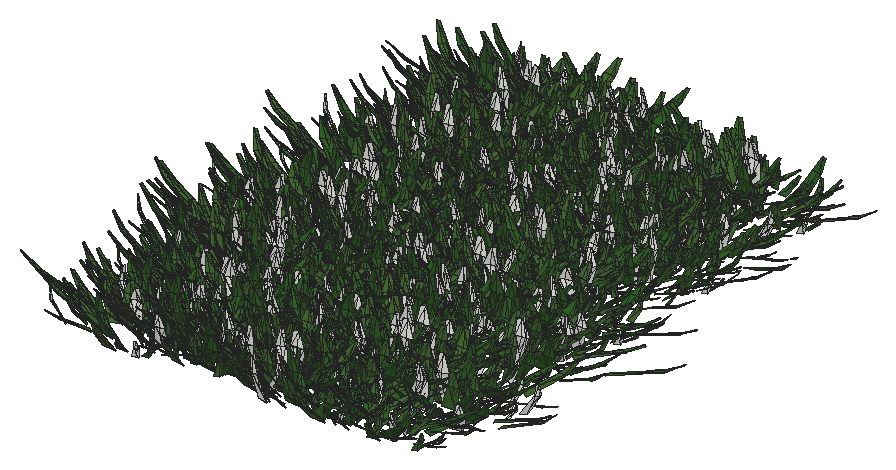
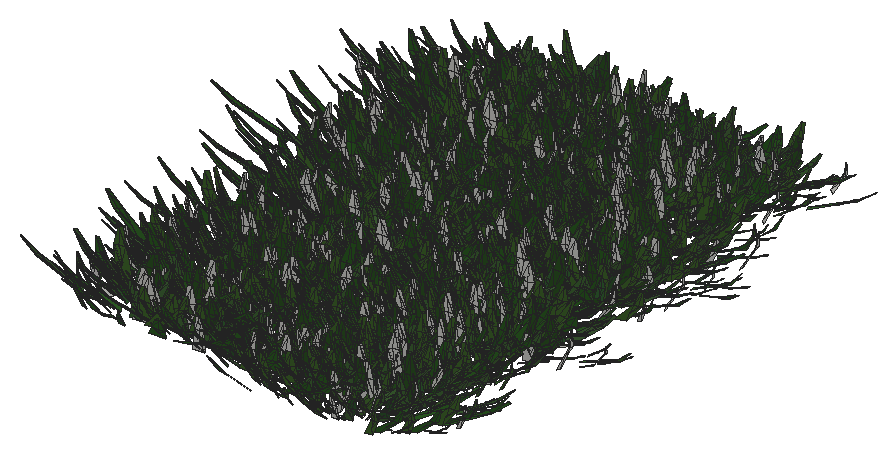
# SketchUp Ruby script. Lengths in inches.
U = 1.inch
M = Sketchup.active_model
def pt(a) = Geom::Point3d.new(a.map { |v| v * U })
def face(e, loops, mat)
  f = e.add_face(loops[0].map { |a| pt(a) })
  loops[1..].each { |l| e.add_face(l.map { |a| pt(a) }).erase! }
  f.material = f.back_material = mat if mat
  f
end
# faces: each face lists its corners as indices into pts; further lists are holes
def faces(e, pts, list, mat = nil) = list.each { |f| face(e, (f[0].is_a?(Array) ? f : [f]).map { |l| l.map { |i| pts[i] } }, mat) }
# xy, xz, yz: faces in a plane at the given z, y or x. An outline is a flat list of corners, or four numbers for a rectangle; further outlines are holes
def ring(l) = l.size == 4 ? [[l[0], l[1]], [l[2], l[1]], [l[2], l[3]], [l[0], l[3]]] : l.each_slice(2).to_a
def flat(e, list, mat, &to3) = list.each { |f| face(e, (f[0].is_a?(Array) ? f : [f]).map { |l| ring(l).map { |u, v| to3.(u, v) } }, mat) }
def xy(e, z, list, mat = nil) = flat(e, list, mat) { |x, y| [x, y, z] }
def xz(e, y, list, mat = nil) = flat(e, list, mat) { |x, z| [x, y, z] }
def yz(e, x, list, mat = nil) = flat(e, list, mat) { |y, z| [x, y, z] }
def lines(e, pts, list) = list.each { |a, b| e.add_line(pt(pts[a]), pt(pts[b])) }
# prism: a flat outline (further loops are holes) pulled along v
def prism(e, loops, v, mat = nil)
  f = face(e, loops, mat); d = Geom::Vector3d.new(v.map { |x| x * U })
  f.pushpull(f.normal.samedirection?(d) ? d.length : -d.length)
end
def box(e, o, s, mat = nil) = prism(e, [[o, [o[0] + s[0], o[1], o[2]], [o[0] + s[0], o[1] + s[1], o[2]], [o[0], o[1] + s[1], o[2]]]], [0, 0, s[2]], mat)
def at(x, y, z, deg = 0) = Geom::Transformation.translation(pt([x, y, z])) * Geom::Transformation.rotation(ORIGIN, Z_AXIS, deg.degrees)
def axes(o, x, y, z) = Geom::Transformation.new([*x, 0, *y, 0, *z, 0, *pt(o).to_a, 1])
def part(name) = M.definitions.add(name)
# library, detail: a bought-in or finely detailed component or shape, given as its bounding box
def library(name, o, s) = part(name).tap { |d| box(d.entities, o, s) }
def detail(e, o, s) = box(e.add_group.entities, o, s)
def put(e, d, t, mat = nil) = e.add_instance(d, t).tap { |i| i.material = mat if mat }
def group(e, t, mat = nil) = e.add_group.tap { |g| g.transformation = t; g.material = mat if mat }.entities
root = M.entities
M.materials.add("Material82").color = [68, 110, 58]
M.materials.add("Material83").color = [48, 90, 38]
M.materials.add("Material84").color = [68, 110, 48]
M.materials.add("Material85").color = [48, 90, 48]
M.materials.add("Material86").color = [58, 110, 58]
M.materials.add("Material87").color = [58, 90, 38]
M.materials.add("Material88").color = [68, 100, 58]
M.materials.add("Material89").color = [48, 100, 38]
c1 = part("grass00")
p = [[-0.6875,0.15,0],[-0.56,0.08,5.52],[-0.04,0.03,2.76],[0.48,-0.02,0],[0.35,-0.02,5.52],[-0.1,-0.14,5.52],
  [-0.12,0.65,8.37],[-0.42,0.65,8.37]]
faces(c1.entities,p,[[0,1,2,3],[3,2,4],[1,5,2],[5,4,2],[1,6,5],[4,5,6],[7,6,1]])
c2 = part("Group16\#1")
put(c2.entities,c1,axes([1.44,-0.61,-0.01],[0.05352,0.12609,0],[-0.10704,0.04543,0.07239],[0.06664,-0.02828,0.11628]),"Material85")
put(c2.entities,c1,axes([0.76,-0.15,-0.01],[0.04676,0.24062,0],[-0.23162,0.04501,0.06642],[0.0652,-0.01267,0.23595]),"Material82")
put(c2.entities,c1,axes([0.79,0.01,-0.01],[-0.00606,0.34651,0],[-0.34381,-0.00602,0.0432],[0.04319,0.00076,0.34386]))
put(c2.entities,c1,axes([1,0.23,-0.01],[-0.07192,0.31144,0],[-0.28722,-0.06632,0.1236],[0.12043,0.02781,0.29478]),"Material84")
put(c2.entities,c1,axes([1.66,0.77,-0.01],[-0.13828,0.29651,0],[-0.21551,-0.1005,0.22471],[0.20365,0.09498,0.23779]),"Material89")
put(c2.entities,c1,axes([0.6875,0.52,-0.01],[-0.18126,0.24051,0],[-0.22746,-0.17142,0.09788],[0.07817,0.05891,0.28481]),"Material84")
put(c2.entities,c1,axes([0.68,0.78,-0.01],[-0.215,0.18688,0],[-0.12385,-0.14248,0.21334],[0.13995,0.16101,0.18878]),"Material82")
put(c2.entities,c1,axes([0.56,1,-0.01],[-0.13756,0.07624,0],[-0.06159,-0.11112,0.0927],[0.04494,0.08108,0.12705]),"Material84")
put(c2.entities,c1,axes([0.2,0.64,-0.01],[-0.23729,0.07254,0],[-0.05711,-0.18681,0.153],[0.04473,0.14632,0.19535]),"Material89")
put(c2.entities,c1,axes([0.0625,0.72,-0.01],[-0.28874,0.02525,0],[-0.02179,-0.24916,0.14647],[0.01276,0.14591,0.25012]),"Material82")
put(c2.entities,c1,axes([-0.08,0.62,-0.01],[-0.34089,-0.04187,0],[0.03255,-0.26504,0.216],[-0.02633,0.21439,0.26703]),"Material89")
put(c2.entities,c1,axes([-0.34,0.98,-0.01],[-0.14314,-0.0493,0],[0.04397,-0.12769,0.06843],[-0.02228,0.0647,0.13505]),"Material89")
put(c2.entities,c1,axes([-0.87,1.45,-0.01],[-0.23488,-0.14114,0],[0.13761,-0.22901,0.06087],[-0.03135,0.05217,0.26717]))
put(c2.entities,c1,axes([-0.72,0.77,-0.01],[-0.14208,-0.13251,0],[0.07209,-0.0773,0.16301],[-0.11118,0.11922,0.1057]),"Material89")
put(c2.entities,c1,axes([-0.62,0.43,-0.01],[-0.14845,-0.21203,0],[0.18654,-0.13061,0.12304],[-0.10079,0.07057,0.22772]),"Material82")
put(c2.entities,c1,axes([-0.68,0.29,-0.01],[-0.13639,-0.32136,0],[0.31723,-0.13464,0.05579],[-0.05136,0.0218,0.34462]),"Material83")
put(c2.entities,c1,axes([-0.64,0.125,-0.01],[-0.0458,-0.23569,0],[0.22124,-0.043,0.08276],[-0.08124,0.01579,0.22538]),"Material86")
put(c2.entities,c1,axes([-1.6,-0.03,-0.01],[0.00576,-0.32897,0],[0.27526,0.00482,0.18018],[-0.18015,-0.00315,0.2753]),"Material84")
put(c2.entities,c1,axes([-1.36,-0.31,-0.01],[0.05718,-0.24765,0],[0.18172,0.04196,0.17267],[-0.16825,-0.03885,0.1865]),"Material89")
put(c2.entities,c1,axes([-1.54,-0.72,-0.01],[0.06537,-0.14017,0],[0.13555,0.06321,0.03939],[-0.0357,-0.01665,0.14956]))
put(c2.entities,c1,axes([-1.19,-0.9,-0.01],[0.09597,-0.12735,0],[0.11214,0.08451,0.07557],[-0.06035,-0.04548,0.14042]),"Material88")
put(c2.entities,c1,axes([-0.47,-0.54,-0.01],[0.11588,-0.10072,0],[0.0618,0.0711,0.12124],[-0.07953,-0.0915,0.0942]))
put(c2.entities,c1,axes([-0.47,-0.84,-0.01],[0.11927,-0.0661,0],[0.06603,0.11913,0.00646],[-0.00313,-0.00565,0.13621]),"Material84")
put(c2.entities,c1,axes([-0.38,-1.24,-0.01],[0.28037,-0.08571,0],[0.0618,0.20215,0.20315],[-0.05939,-0.19428,0.21139]),"Material88")
put(c2.entities,c1,axes([-0.06,-0.66,-0.01],[0.22719,-0.01987,0],[0.01247,0.14255,0.17758],[-0.01547,-0.17691,0.1431]),"Material87")
put(c2.entities,c1,axes([0.11,-0.89,-0.01],[0.14882,0.01828,0],[-0.01058,0.08611,0.12229],[0.01491,-0.12138,0.08676]),"Material85")
put(c2.entities,c1,axes([0.25,-0.72,-0.01],[0.20481,0.07053,0],[-0.06206,0.18022,0.10291],[0.03351,-0.0973,0.1906]),"Material85")
put(c2.entities,c1,axes([0.85,-1.42,-0.01],[0.16481,0.09904,0],[-0.09472,0.15762,0.05616],[0.02893,-0.04814,0.18389]),"Material84")
put(c2.entities,c1,axes([1.01,-1.09,-0.01],[0.21858,0.20385,0],[-0.17495,0.1876,0.15339],[0.10462,-0.11218,0.25652]),"Material89")
put(c2.entities,c1,axes([1.01,-0.71,-0.01],[0.08733,0.12473,0],[-0.06445,0.04512,0.13037],[0.1068,-0.07477,0.07867]),"Material85")
c3 = part("Group15\#1")
put(c3.entities,c2,at(0,0,0))
c4 = part("3darcstudiotree_grass00\#1")
put(c4.entities,c3,at(0,0,0))
put(root,c4,axes([655.18,1033.95,-29.74],[4.10302,-0.30694,0],[0.8385,1.74326,-0.00778],[0.00611,0.0127,1.42033]))
put(root,c4,axes([655.57,1017.02,-29.74],[-2.0309,1.41107,0],[-3.96455,-0.88745,-0.03094],[-0.10652,-0.02384,1.35284]))
put(root,c4,axes([655.39,1018.32,-29.74],[3.97679,-0.10087,0],[0.2922,1.7917,-0.04097],[0.01281,0.07857,1.66267]))
put(root,c4,axes([656.06,1024.5,-29.74],[2.96266,-0.9536,0],[2.21709,1.07131,-0.03627],[0.16479,0.07963,1.88825]))
put(root,c4,axes([657.22,1009.61,-29.74],[-2.64678,-1.36079,0],[3.05956,-0.92555,-0.03114],[0.16031,-0.04849,1.87535]))
put(root,c4,axes([656.63,1048.64,-29.74],[2.77032,-1.11765,0],[2.79461,1.07735,-0.00015],[0.00071,0.00027,1.98495]))
put(root,c4,axes([655.75,1012.55,-29.74],[1.36747,1.27936,0],[-3.91602,0.651,-0.04214],[-0.23603,0.03924,1.93625]))
put(root,c4,axes([657.62,1031.41,-29.74],[-0.46652,-1.63259,0],[3.80254,-0.169,-0.02839],[0.12966,-0.00576,1.31807]))
put(root,c4,axes([657.72,1038.09,-29.74],[-2.24585,-1.17679,0],[2.75058,-0.81643,-0.02546],[0.1532,-0.04547,1.94365]))
put(root,c4,axes([658.32,1047.5,-29.74],[-3.1613,-1.38915,0],[3.20855,-1.13563,-0.02493],[0.08224,-0.02911,1.43253]))
put(root,c4,axes([658.0625,1051.55,-29.74],[-4.11217,-0.39094,0],[0.86082,-1.40827,-0.01967],[0.02693,-0.04406,1.60841]))
put(root,c4,axes([657.42,1021.11,-29.74],[-2.52022,1.35688,0],[-2.71694,-0.78485,-0.02032],[-0.10759,-0.03108,1.65635]))
put(root,c4,axes([658.07,1001.24,-29.74],[-3.93546,0.24929,0],[-0.63824,-1.56709,-0.04907],[-0.04216,-0.10352,1.63442]))
put(root,c4,axes([657.66,1040.7,-29.74],[1.48309,-1.18944,0],[3.17184,0.61511,-0.04022],[0.27217,0.05278,1.99791]))
put(root,c4,axes([656.82,998.44,-29.74],[-0.1961,1.67231,0],[-3.9427,-0.07191,-0.00948],[-0.04368,-0.0008,1.36423]))
put(root,c4,axes([658.58,1042.42,-29.74],[-1.75334,-1.53625,0],[3.78301,-0.67151,-0.04331],[0.23983,-0.04257,1.88835]))
put(root,c4,axes([658.72,1045.07,-29.74],[-1.47837,-1.71881,0],[3.4357,-0.4596,-0.01224],[0.08437,-0.01129,1.97883]))
put(root,c4,axes([656.95,1022.94,-29.74],[0.89151,1.73156,0],[-4.53511,0.36315,-0.02679],[-0.1364,0.01092,1.80175]))
put(root,c4,axes([657.53,1002.9,-29.74],[3.29656,-0.16392,0],[0.52833,1.6525,-0.05027],[0.03097,0.09687,1.55905]))
put(root,c4,axes([656.95,1035.78,-29.74],[1.8424,1.14237,0],[-3.65624,0.91712,-0.00074],[-0.00371,0.00093,1.93092]))
put(root,c4,axes([658.37,1014.64,-29.74],[2.92684,-0.73502,0],[1.91435,1.18558,-0.0345],[0.12831,0.07947,1.8497]))
put(root,c4,axes([658.57,1005.96,-29.74],[0.10092,1.39888,0],[-4.08431,0.04583,-0.02239],[-0.13434,0.00151,1.83839]))
put(root,c4,axes([658.65,1029.15,-29.74],[-0.46714,1.44095,0],[-4.49775,-0.22678,-0.0277],[-0.15196,-0.00766,1.87956]))
put(root,c4,axes([660.68,1019.2,-29.74],[-2.63576,-1.28026,0],[3.53005,-1.13032,-0.02494],[0.11128,-0.03563,1.95866]))
put(root,c4,axes([660.64,1053.33,-29.74],[-3.99047,-0.40873,0],[1.06863,-1.62266,-0.00758],[0.01027,-0.0156,1.7185]))
put(root,c4,axes([660.37,1029.42,-29.74],[-0.06008,-1.38054,0],[4.09358,-0.02771,-0.0405],[0.24938,-0.00169,1.89003]))
put(root,c4,axes([660.76,1036.51,-29.74],[-1.38876,-1.54798,0],[3.56891,-0.49797,-0.03351],[0.18812,-0.02625,1.68972]))
put(root,c4,axes([661.375,1046.76,-29.74],[-0.94917,-1.78727,0],[4.28932,-0.35429,-0.02019],[0.10216,-0.00844,1.69814]))
put(root,c4,axes([661.2,1052.08,-29.74],[-0.90047,-1.75818,0],[4.05941,-0.32336,-0.03802],[0.21461,-0.0171,1.78771]))
put(root,c4,axes([661.53,1021.48,-29.74],[-2.86404,-0.64452,0],[1.81455,-1.25407,-0.04344],[0.15373,-0.10625,1.9596]))
put(root,c4,axes([661.78,1009.37,-29.74],[-1.66133,-1.5225,0],[4.09169,-0.6944,-0.04688],[0.21591,-0.03664,1.67419]))
put(root,c4,axes([661.71,1015.88,-29.74],[-3.61877,0.99301,0],[-2.17277,-1.23149,-0.01001],[-0.02667,-0.01512,1.32974]))
put(root,c4,axes([662.72,1027.38,-29.74],[-0.34586,-1.45501,0],[4.09876,-0.15153,-0.00863],[0.04038,-0.00149,1.44957]))
put(root,c4,axes([663.3,1014.23,-29.74],[-1.55676,-1.64059,0],[4.33421,-0.63965,-0.05081],[0.20494,-0.03024,1.49393]))
put(root,c4,axes([661.89,1024.86,-29.74],[4.37611,-0.60729,0],[1.31361,1.47222,-0.0057],[0.0109,0.01221,1.70987]))
put(root,c4,axes([663.38,1042.79,-29.74],[-0.47275,-1.4969,0],[4.46074,-0.21911,-0.06365],[0.35527,-0.01745,1.89522]))
put(root,c4,axes([662.97,1038.82,-29.74],[2.20658,-1.37183,0],[2.86337,0.71632,-0.01781],[0.08885,0.02223,1.50117]))
put(root,c4,axes([662.61,1049.89,-29.74],[3.60935,-0.56815,0],[1.37625,1.35979,-0.02611],[0.05001,0.04941,1.43783]))
put(root,c4,axes([663.8,1002.8,-29.74],[-3.927,-0.17218,0],[0.45946,-1.62986,-0.05312],[0.03146,-0.11159,1.67036]))
put(root,c4,axes([662.71,1000.79,-29.74],[4.2823,-0.66393,0],[1.32307,1.32724,-0.00849],[0.02062,0.02068,1.79934]))
put(root,c4,axes([663.99,1033.72,-29.74],[0.52677,-1.54843,0],[3.37532,0.17859,-0.00096],[0.0064,0.00034,1.71349]))
put(root,c4,axes([663.97,1031.74,-29.74],[-3.78642,0.03695,0],[-0.11198,-1.78455,-0.01248],[-0.00125,-0.01991,1.37214]))
put(root,c4,axes([664.18,1045.21,-29.74],[-3.50363,0.54877,0],[-1.37004,-1.36042,-0.04199],[-0.09387,-0.09321,1.68502]))
put(root,c4,axes([664.02,1023.08,-29.74],[-3.78815,1.05417,0],[-2.08305,-1.1642,0],[-0.00001,-0.00001,1.91868]))
put(root,c4,axes([663.28,999.37,-29.74],[3.14187,0.39177,0],[-1.17778,1.46906,-0.04459],[-0.07661,0.09555,1.66873]))
put(root,c4,axes([664.48,1040.2,-29.74],[-4.05008,0.95977,0],[-1.76425,-1.15789,-0.02116],[-0.06339,-0.0416,1.49339]))
put(root,c4,axes([664.18,1005.88,-29.74],[-2.14427,1.00131,0],[-3.09998,-1.03248,-0.03207],[-0.1604,-0.05342,1.99077]))
put(root,c4,axes([664.36,1007.9,-29.74],[-3.03453,1.36043,0],[-3.50876,-1.21725,-0.06393],[-0.1925,-0.06678,1.40472]))
put(root,c4,axes([664.19,1011.48,-29.74],[4.55933,-0.17295,0],[0.45061,1.84755,-0.06081],[0.02387,0.09789,1.44654]))
put(root,c4,axes([666.05,1026.73,-29.74],[-0.03672,-1.35909,0],[4.67682,-0.01965,-0.05216],[0.20276,-0.00085,1.36288]))
put(root,c4,axes([666.16,1012.2,-29.74],[0.13892,-1.80916,0],[4.0915,0.04886,-0.01983],[0.09749,0.00116,1.50947]))
put(root,c4,axes([666.41,1045.11,-29.74],[-0.70107,-1.67232,0],[4.13597,-0.26967,-0.0168],[0.0818,-0.00533,1.55067]))
put(root,c4,axes([666.55,1016.1875,-29.74],[-3.75519,-1.14447,0],[2.68213,-1.36874,-0.06061],[0.1619,-0.08262,1.43628]))
put(root,c4,axes([666.08,1028.91,-29.74],[-0.54027,-1.6401,0],[3.32557,-0.17038,-0.04034],[0.23473,-0.01203,1.47504]))
put(root,c4,axes([666.3125,1024.72,-29.74],[-3.58356,0.46021,0],[-1.0679,-1.2933,-0.04555],[-0.08783,-0.10637,1.60995]))
put(root,c4,axes([666.78,1002.92,-29.74],[-3.8661,0.57248,0],[-1.34665,-1.41442,-0.01194],[-0.02505,-0.02631,1.71307]))
put(root,c4,axes([666.98,1010.36,-29.74],[-3.59396,1.08002,0],[-2.30452,-1.19271,-0.04347],[-0.15376,-0.07958,1.66314]))
put(root,c4,axes([667.76,999.57,-29.74],[-3.24117,-0.71309,0],[1.62667,-1.14993,-0.00653],[0.01841,-0.01301,1.4475]))
put(root,c4,axes([668.11,1043.23,-29.74],[-3.07387,-1.37226,0],[2.57369,-0.89663,-0.00245],[0.01347,-0.00469,1.8862]))
put(root,c4,axes([666.375,1049.15,-29.74],[0.39811,1.50692,0],[-3.94981,0.16229,-0.02993],[-0.16157,0.00664,1.61572]))
put(root,c4,axes([666.47,1022.58,-29.74],[-0.46786,1.28327,0],[-3.81344,-0.21623,-0.00494],[-0.02392,-0.00136,1.4129]))
put(root,c4,axes([668.26,1005.55,-29.74],[0.52643,-1.67667,0],[4.29673,0.20982,-0.00236],[0.01155,0.00056,1.5989]))
put(root,c4,axes([666.98,1046.66,-29.74],[3.86987,-0.34459,0],[0.79622,1.39073,-0.03599],[0.03867,0.06754,1.32194]))
put(root,c4,axes([668.06,1031.85,-29.74],[-3.89357,0.61481,0],[-1.50479,-1.48217,-0.00598],[-0.01246,-0.01228,1.70205]))
put(root,c4,axes([667.21,1007.16,-29.74],[4.26757,-0.1267,0],[0.26808,1.40432,-0.02417],[0.01226,0.06424,1.80918]))
put(root,c4,axes([667.26,1050.8125,-29.74],[0.18137,1.61713,0],[-3.86456,0.06741,-0.03464],[-0.18684,0.00326,1.56527]))
put(root,c4,axes([667.04,1052.95,-29.74],[2.68425,0.98126,0],[-3.08103,1.31083,-0.0132],[-0.04194,0.01784,1.58767]))
put(root,c4,axes([668.82,1018.3,-29.74],[-4.03193,0.12785,0],[-0.33897,-1.66251,-0.04274],[-0.01416,-0.06944,1.31001]))
put(root,c4,axes([669.16,1033.54,-29.74],[-2.54975,-1.13663,0],[2.74994,-0.95943,-0.02762],[0.1264,-0.0441,1.68176]))
put(root,c4,axes([667.44,1020.33,-29.74],[2.51292,1.08795,0],[-3.26468,1.1728,-0.05824],[-0.20485,0.07359,1.57486]))
put(root,c4,axes([668.61,1037.86,-29.74],[2.12492,-1.52639,0],[3.32667,0.72027,-0.02765],[0.13101,0.02837,1.53783]))
put(root,c4,axes([667.9375,1001.04,-29.74],[2.57949,0.81299,0],[-2.19489,1.0831,-0.04441],[-0.18645,0.09201,1.772]))
put(root,c4,axes([668.86,1040.1,-29.74],[2.26224,-1.2031,0],[3.43735,1.00525,-0.03781],[0.13632,0.03987,1.4396]))
put(root,c4,axes([668.03,1035.7,-29.74],[0.64746,1.71828,0],[-3.59,0.21039,-0.03328],[-0.18561,0.01088,1.53387]))
put(root,c4,axes([669.1,1013.91,-29.74],[1.65411,1.32331,0],[-4.02119,0.78176,-0.01549],[-0.05875,0.01142,1.42146]))
put(root,c4,axes([671.84,1000.57,-29.74],[-1.99996,-1.21087,0],[3.64955,-0.93751,-0.00487],[0.02184,-0.00561,1.74651]))
put(root,c4,axes([671.62,1049.92,-29.74],[-4.08637,0.5893,0],[-1.1512,-1.24155,-0.04181],[-0.0785,-0.08466,1.37365]))
put(root,c4,axes([671.89,1033.33,-29.74],[0.94723,-1.59052,0],[4.2139,0.39031,-0.04288],[0.2193,0.02031,1.70449]))
put(root,c4,axes([672.09,1003.34,-29.74],[0.76825,-1.34447,0],[4.07723,0.36235,-0.02216],[0.10533,0.00936,1.52603]))
put(root,c4,axes([672.72,1039.85,-29.74],[-4.28344,0.1007,0],[-0.25434,-1.68266,-0.00226],[-0.00079,-0.00521,1.87745]))
put(root,c4,axes([672.39,1044.92,-29.74],[1.6756,-1.36696,0],[3.5262,0.67226,-0.03335],[0.16368,0.0312,1.60043]))
put(root,c4,axes([673.01,1012.25,-29.74],[-0.47602,-1.5827,0],[4.1601,-0.1946,-0.02638],[0.12052,-0.00564,1.44452]))
put(root,c4,axes([672.05,1036.29,-29.74],[4.15464,-0.59094,0],[1.53872,1.68251,-0.06016],[0.09162,0.10018,1.52593]))
put(root,c4,axes([672.3,1020.84,-29.74],[-1.67139,1.30839,0],[-3.46219,-0.68786,-0.03585],[-0.17478,-0.03472,1.58646]))
put(root,c4,axes([672.89,1027.42,-29.74],[-3.50073,0.942,0],[-2.16331,-1.25037,-0.04776],[-0.1565,-0.09046,1.6727]))
put(root,c4,axes([672.24,1019.13,-29.74],[3.80678,-0.63656,0],[1.53404,1.42681,-0.02583],[0.05775,0.05372,1.68703]))
put(root,c4,axes([672.65,1047.1875,-29.74],[4.59121,-0.45029,0],[0.84969,1.34743,-0.00031],[0.00049,0.00078,1.72722]))
put(root,c4,axes([673.2,1013.65,-29.74],[3.46257,-0.87441,0],[2.25752,1.39035,-0.00312],[0.00811,0.00499,1.51309]))
put(root,c4,axes([672.82,1016.7,-29.74],[4.45522,-0.42871,0],[0.88291,1.42703,-0.01844],[0.02851,0.04608,1.82062]))
put(root,c4,axes([673.77,1038.17,-29.74],[2.11135,-1.17998,0],[3.12805,0.87051,-0.01427],[0.05324,0.01482,1.30992]))
put(root,c4,axes([673.86,1007.3125,-29.74],[2.70908,-1.29001,0],[3.26836,1.0675,-0.01649],[0.07179,0.02345,1.79785]))
put(root,c4,axes([674.59,1030.05,-29.74],[-1.99014,-1.36063,0],[3.61455,-0.82226,-0.05686],[0.20653,-0.04698,1.31145]))
put(root,c4,axes([674.58,1051.25,-29.74],[-4.63629,0.17249,0],[-0.31305,-1.3087,-0.02738],[-0.01684,-0.0704,1.63584]))
put(root,c4,axes([674.26,1025.35,-29.74],[1.2093,-1.57862,0],[4.10109,0.48862,-0.03916],[0.21176,0.02523,1.81408]))
put(root,c4,axes([672.8,1031.42,-29.74],[2.22707,1.32751,0],[-3.83725,1.00121,-0.02773],[-0.10131,0.02643,1.51065]))
put(root,c4,axes([673.59,1042.79,-29.74],[0.32393,1.2922,0],[-3.8703,0.1509,-0.01511],[-0.10076,0.00393,1.95375]))
put(root,c4,axes([673.78,1004.77,-29.74],[3.29328,0.79365,0],[-2.38723,1.54066,-0.04231],[-0.12354,0.07973,1.92144]))
put(root,c4,axes([675.49,1010.29,-29.74],[-4.33123,0.18779,0],[-0.372,-1.33439,-0.04038],[-0.02759,-0.09898,1.5952]))
put(root,c4,axes([675.14,999.125,-29.74],[-2.43738,1.19248,0],[-2.72185,-0.86527,-0.02131],[-0.12,-0.03815,1.8955]))
put(root,c4,axes([675.09,1023.49,-29.74],[-1.08989,1.28976,0],[-3.11811,-0.40981,-0.02384],[-0.1661,-0.02183,1.80943]))
put(root,c4,axes([676.99,1031.61,-29.74],[0.31301,-1.31124,0],[3.5948,0.13346,-0.01523],[0.11152,0.00414,1.99019]))
put(root,c4,axes([677.54,1004.77,-29.74],[-3.40339,-1.11564,0],[2.13204,-1.01156,-0.01701],[0.08509,-0.04037,1.95649]))
put(root,c4,axes([677.9,1017.9,-29.74],[-3.55731,-0.39699,0],[0.91028,-1.26863,-0.03071],[0.04629,-0.06451,1.38702]))
put(root,c4,axes([677.41,1012.59,-29.74],[1.53941,-1.17663,0],[3.76142,0.76538,-0.04957],[0.23972,0.04878,1.72633]))
put(root,c4,axes([677.88,1043.03,-29.74],[-0.12409,-1.44715,0],[3.33282,-0.04445,-0.02047],[0.13634,-0.00182,1.66543]))
put(root,c4,axes([677.61,1010.14,-29.74],[1.91221,-1.68967,0],[4.00415,0.70478,-0.04062],[0.20203,0.03556,1.79015]))
put(root,c4,axes([677.54,1040.36,-29.74],[-2.75564,1.16599,0],[-3.11928,-1.14656,-0.00031],[-0.00116,-0.00043,1.61707]))
put(root,c4,axes([677.47,1016.95,-29.74],[3.14616,-0.46124,0],[1.36147,1.44435,-0.02775],[0.06352,0.06739,1.92398]))
put(root,c4,axes([678.87,1025.6,-29.74],[-0.59398,-1.49967,0],[3.68059,-0.22673,-0.04759],[0.22724,-0.014,1.34947]))
put(root,c4,axes([679.42,1038.39,-29.74],[-1.90322,-1.23489,0],[2.93996,-0.70472,-0.04312],[0.27444,-0.06578,1.92045]))
put(root,c4,axes([679.6,1047.59,-29.74],[-2.12705,-1.09895,0],[2.82257,-0.84968,-0.04177],[0.17079,-0.05141,1.36919]))
put(root,c4,axes([679.71,1014.16,-29.74],[1.44153,-1.60776,0],[3.23959,0.45176,-0.02361],[0.11408,0.01591,1.32009]))
put(root,c4,axes([678.75,1045.27,-29.74],[1.45904,1.69634,0],[-4.12454,0.55175,-0.04327],[-0.22093,0.02955,1.7601]))
put(root,c4,axes([678.95,1033.61,-29.74],[0.41076,1.77313,0],[-3.60416,0.12986,-0.02215],[-0.11578,0.00417,1.42375]))
put(root,c4,axes([680.13,1036.79,-29.74],[0.96466,-1.81909,0],[3.32191,0.27398,-0.01603],[0.09156,0.00755,1.48463]))
put(root,c4,axes([679.14,1008.52,-29.74],[-0.86085,1.83609,0],[-4.61027,-0.33618,-0.00297],[-0.01572,-0.00115,1.8915]))
put(root,c4,axes([679.44,1050.66,-29.74],[3.95759,-0.11816,0],[0.2883,1.50178,-0.04662],[0.02067,0.10765,1.68074]))
put(root,c4,axes([679.59,1049.83,-29.74],[-0.65253,1.4678,0],[-3.82967,-0.26479,-0.02601],[-0.14603,-0.0101,1.66111]))
put(root,c4,axes([679.07,1001.16,-29.74],[2.91821,1.08875,0],[-2.82314,1.17688,-0.00432],[-0.01382,0.00576,1.43292]))
put(root,c4,axes([680.33,1029.41,-29.74],[3.48292,-0.82099,0],[2.25154,1.48559,-0.05659],[0.14545,0.09597,1.64805]))
put(root,c4,axes([679.78,998.86,-29.74],[4.39717,0.52423,0],[-1.00944,1.31686,-0.04581],[-0.07981,0.10411,1.57403]))
put(root,c4,axes([679.76,1027.59,-29.74],[3.42406,1.01361,0],[-2.506,1.31662,-0.02233],[-0.08435,0.04432,1.9689]))
put(root,c4,axes([680.47,1020.98,-29.74],[-2.64058,1.54622,0],[-3.55505,-0.94424,-0.0002],[-0.001,-0.00026,1.96126]))
put(root,c4,axes([680.8125,1022.34,-29.74],[4.33275,-0.34682,0],[0.77843,1.5125,-0.04034],[0.04996,0.09707,1.82611]))
put(root,c4,axes([682.63,1047.06,-29.74],[-3.32048,-0.89448,0],[2.67505,-1.54445,-0.03279],[0.08824,-0.05095,1.69581]))
put(root,c4,axes([680.78,1004.125,-29.74],[3.65442,0.79234,0],[-1.92667,1.38205,-0.0244],[-0.05154,0.03697,1.31386]))
put(root,c4,axes([683.2,1023.16,-29.74],[-4.47242,-0.43212,0],[1.12449,-1.81009,-0.038],[0.04833,-0.0778,1.89315]))
put(root,c4,axes([683.17,1040.74,-29.74],[3.41982,0.22152,0],[-0.58321,1.40029,-0.00501],[-0.00425,0.0102,1.40942]))
put(root,c4,axes([683.11,1050.02,-29.74],[0.62564,1.8219,0],[-4.46763,0.23861,-0.03426],[-0.17796,0.0095,1.77113]))
put(root,c4,axes([683.8125,1034.15,-29.74],[3.06207,-0.55792,0],[1.42852,1.21938,-0.0238],[0.07482,0.06387,1.9133]))
put(root,c4,axes([684.28,1016.52,-29.74],[2.42149,-1.19086,0],[3.28427,1.03866,-0.04277],[0.16953,0.05361,1.60323]))
put(root,c4,axes([685.24,1005.76,-29.74],[-4.5051,-0.1347,0],[0.33952,-1.76605,-0.05601],[0.0175,-0.09103,1.39118]))
put(root,c4,axes([685.37,1009.92,-29.74],[-3.05686,-1.19982,0],[3.00062,-1.189,-0.05331],[0.20258,-0.08027,1.71744]))
put(root,c4,axes([685.36,1007.22,-29.74],[0.58993,-1.49665,0],[4.0908,0.25078,-0.01704],[0.09795,0.00601,1.80481]))
put(root,c4,axes([683.91,1002.86,-29.74],[0.93986,1.81776,0],[-4.11362,0.3308,-0.03996],[-0.17618,0.01417,1.416]))
put(root,c4,axes([683.92,1031.26,-29.74],[1.86,1.67689,0],[-3.22779,0.55683,-0.02724],[-0.14202,0.0245,1.50258]))
put(root,c4,axes([684.2,1014.91,-29.74],[3.80375,0.01195,0],[-0.02861,1.41659,-0.01492],[-0.00081,0.04025,1.84219]))
put(root,c4,axes([684.23,999.27,-29.74],[3.00521,0.63807,0],[-1.62064,1.18715,-0.02125],[-0.05194,0.03805,1.32121]))
put(root,c4,axes([685.1,1050.73,-29.74],[-2.17573,1.65884,0],[-3.97455,-0.81077,-0.04288],[-0.19169,-0.0391,1.68813]))
put(root,c4,axes([685.27,1025.03,-29.74],[-1.91722,1.31385,0],[-4.0358,-0.91594,-0.03664],[-0.12047,-0.02734,1.3241]))
put(root,c4,axes([685.02,1038.56,-29.74],[2.76774,0.7917,0],[-1.93345,1.05126,-0.02439],[-0.09329,0.05072,1.60766]))
put(root,c4,axes([685.5,1018.54,-29.74],[4.38931,-0.45982,0],[1.18067,1.75286,-0.06211],[0.07411,0.11002,1.60192]))
put(root,c4,axes([686.27,1042.83,-29.74],[1.79387,-1.26785,0],[3.18419,0.70071,-0.05199],[0.23586,0.0519,1.41973]))
put(root,c4,axes([685.96,1036.38,-29.74],[-1.97144,1.08801,0],[-3.33394,-0.93955,-0.01309],[-0.05439,-0.01533,1.56859]))
